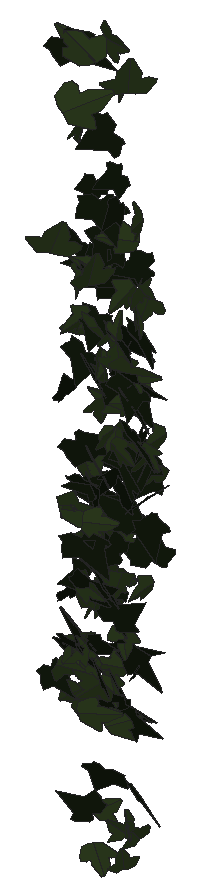
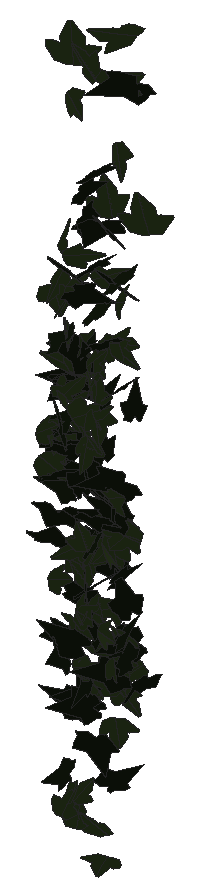
# SketchUp Ruby script. Lengths in inches.
U = 1.inch
M = Sketchup.active_model
def pt(a) = Geom::Point3d.new(a.map { |v| v * U })
def face(e, loops, mat)
  f = e.add_face(loops[0].map { |a| pt(a) })
  loops[1..].each { |l| e.add_face(l.map { |a| pt(a) }).erase! }
  f.material = f.back_material = mat if mat
  f
end
# faces: each face lists its corners as indices into pts; further lists are holes
def faces(e, pts, list, mat = nil) = list.each { |f| face(e, (f[0].is_a?(Array) ? f : [f]).map { |l| l.map { |i| pts[i] } }, mat) }
# xy, xz, yz: faces in a plane at the given z, y or x. An outline is a flat list of corners, or four numbers for a rectangle; further outlines are holes
def ring(l) = l.size == 4 ? [[l[0], l[1]], [l[2], l[1]], [l[2], l[3]], [l[0], l[3]]] : l.each_slice(2).to_a
def flat(e, list, mat, &to3) = list.each { |f| face(e, (f[0].is_a?(Array) ? f : [f]).map { |l| ring(l).map { |u, v| to3.(u, v) } }, mat) }
def xy(e, z, list, mat = nil) = flat(e, list, mat) { |x, y| [x, y, z] }
def xz(e, y, list, mat = nil) = flat(e, list, mat) { |x, z| [x, y, z] }
def yz(e, x, list, mat = nil) = flat(e, list, mat) { |y, z| [x, y, z] }
def lines(e, pts, list) = list.each { |a, b| e.add_line(pt(pts[a]), pt(pts[b])) }
# prism: a flat outline (further loops are holes) pulled along v
def prism(e, loops, v, mat = nil)
  f = face(e, loops, mat); d = Geom::Vector3d.new(v.map { |x| x * U })
  f.pushpull(f.normal.samedirection?(d) ? d.length : -d.length)
end
def box(e, o, s, mat = nil) = prism(e, [[o, [o[0] + s[0], o[1], o[2]], [o[0] + s[0], o[1] + s[1], o[2]], [o[0], o[1] + s[1], o[2]]]], [0, 0, s[2]], mat)
def at(x, y, z, deg = 0) = Geom::Transformation.translation(pt([x, y, z])) * Geom::Transformation.rotation(ORIGIN, Z_AXIS, deg.degrees)
def axes(o, x, y, z) = Geom::Transformation.new([*x, 0, *y, 0, *z, 0, *pt(o).to_a, 1])
def part(name) = M.definitions.add(name)
# library, detail: a bought-in or finely detailed component or shape, given as its bounding box
def library(name, o, s) = part(name).tap { |d| box(d.entities, o, s) }
def detail(e, o, s) = box(e.add_group.entities, o, s)
def put(e, d, t, mat = nil) = e.add_instance(d, t).tap { |i| i.material = mat if mat }
def group(e, t, mat = nil) = e.add_group.tap { |g| g.transformation = t; g.material = mat if mat }.entities
root = M.entities
M.materials.add("1026 AP 7946 SUNNY SIDE UP").color = [254, 231, 186]
M.materials.add("efeu1").color = [18, 25, 13]
M.materials.add("efeu2").color = [43, 57, 29]
c1 = part("ivyleaf_10")
p = [[0,0.5,-0.03],[-0.0625,2.02,-0.43],[-0.19,2.01,-0.46],[-0.54,1.05,-0.29],[-0.52,0.625,-0.18],[-0.83,0.76,-0.28],
  [-1.16,0.64,-0.33],[-1.15,0.33,-0.24],[-0.77,-0.39,0.02],[-0.3,-0.51,0.16],[0.04,-0.48,0.23],[-0.02,2.01,-0.4375],
  [-0.06,2.01,-0.43],[0.04,-0.49,0.23],[0.67,-0.49,0.14],[1.38,0.36,-0.2],[1.375,0.51,-0.24],[0.81,0.65,-0.19],
  [0.62,0.59,-0.15],[0.6,1.09,-0.28],[0.5,1.23,-0.31]]
faces(c1.entities,p,[[0,1,2,3,4,5,6,7,8,9,10],[11,12,0,13,14,15,16,17,18,19,20]],"efeu2")
c2 = part("ivyleaf_9")
p = [[1.54,2.16,1.25],[1.36,2.04,1.19],[-0.21,0.99,0.68],[-0.71,1.11,0.82],[-0.85,0.86,0.67],[-0.8,0.17,0.21],
  [-0.9,-0.01,0.1],[-0.67,-0.16,-0.02],[-0.08,-0.08,-0.05],[-0.03,-0.6,-0.4],[0.65,-0.88,-0.66],[0.83,-0.6,-0.49],
  [1.29,-0.42,-0.43],[1.8125,-0.07,-0.26],[1.21,0.44,0.15]]
faces(c2.entities,p,[[0,1,2,3,4,5,6,7,8,9,10,11,12,13,14]],"efeu1")
put(root,c1,axes([111.49,209.65,262.91],[-0.17375,-0.32185,-0.02419],[-0.02548,-0.01732,0.35033],[-0.50659,0.11126,-0.00932]),"1026 AP 7946 SUNNY SIDE UP")
put(root,c1,axes([111.22,209.35,266.96],[0.25556,0.02321,-0.35537],[0.36802,0.27334,0.1341],[0.4004,-0.26605,0.10356]),"1026 AP 7946 SUNNY SIDE UP")
put(root,c1,axes([110.24,209.98,263.08],[-0.38999,-0.21873,0.04558],[0.02966,0.04722,0.34015],[-0.35003,0.2477,-0.02196]),"1026 AP 7946 SUNNY SIDE UP")
put(root,c1,axes([111.14,209.96,252.59],[0.10276,-0.01725,-0.25564],[0.3866,0.04274,0.06392],[0.05831,-0.25293,0.02671]),"1026 AP 7946 SUNNY SIDE UP")
put(root,c2,axes([111.08,210.48,253.16],[-0.01812,-0.07901,0.2553],[0.02696,-0.2482,-0.082],[0.40878,0.01287,0.01673]),"1026 AP 7946 SUNNY SIDE UP")
put(root,c2,axes([110.69,210.51,255.03],[-0.04185,-0.03352,0.27533],[0.32226,-0.17708,-0.00289],[0.2753,0.20219,0.04524]),"1026 AP 7946 SUNNY SIDE UP")
put(root,c1,axes([110.55,210.51,255.15],[-0.00463,0.00813,0.27853],[0.41593,-0.05615,0.00438],[0.08846,0.26444,-0.00601]),"1026 AP 7946 SUNNY SIDE UP")
put(root,c2,axes([111.0625,210.62,255.24],[0.27088,-0.15391,-0.13249],[0.17626,-0.06532,0.23644],[-0.26045,-0.20427,0.02222]),"1026 AP 7946 SUNNY SIDE UP")
put(root,c2,axes([110.75,210.56,249.9],[0.01042,0.03582,0.25038],[-0.3547,-0.09489,0.02021],[0.15218,-0.22363,0.02995]),"1026 AP 7946 SUNNY SIDE UP")
put(root,c1,axes([110.4,210.61,253.59],[0.33866,-0.13345,-0.08962],[-0.13366,0.02596,-0.25993],[0.21109,0.23054,-0.02079]),"1026 AP 7946 SUNNY SIDE UP")
put(root,c2,axes([110.72,210.8,257.79],[-0.03519,-0.08172,0.27107],[0.08662,-0.26045,-0.0799],[0.4252,0.0463,0.03871]),"1026 AP 7946 SUNNY SIDE UP")
put(root,c2,axes([110.48,210.62,256.1],[-0.08192,-0.17821,-0.20654],[0.1772,0.16968,-0.1855],[0.38144,-0.1171,0.04182]),"1026 AP 7946 SUNNY SIDE UP")
put(root,c1,axes([111.62,210.72,266.97],[-0.3525,-0.27041,-0.0294],[-0.05405,-0.0065,0.36109],[-0.42387,0.22571,-0.0216]),"1026 AP 7946 SUNNY SIDE UP")
put(root,c2,axes([109.98,210.64,253.55],[0.39055,-0.0623,0.07124],[0.09668,-0.03946,-0.26302],[0.11043,0.25489,-0.02169]),"1026 AP 7946 SUNNY SIDE UP")
put(root,c1,axes([111.48,210.74,248.8125],[-0.15422,-0.19699,-0.07207],[-0.06317,-0.05682,0.22612],[-0.32197,0.1055,-0.00984]),"1026 AP 7946 SUNNY SIDE UP")
put(root,c2,axes([111.04,210.66,250.9],[0.22813,0.10021,-0.17766],[-0.21129,-0.10944,-0.18201],[-0.23282,0.19751,-0.0089]),"1026 AP 7946 SUNNY SIDE UP")
put(root,c1,axes([111.39,210.84,249.52],[-0.12943,-0.13186,-0.17606],[-0.1636,-0.13511,0.15892],[-0.29632,0.13219,-0.01084]),"1026 AP 7946 SUNNY SIDE UP")
put(root,c2,axes([109.67,210.66,252.8],[0.08125,-0.16649,-0.18844],[-0.06214,0.17793,-0.17823],[0.38281,0.06422,0.01107]),"1026 AP 7946 SUNNY SIDE UP")
put(root,c2,axes([110.33,210.92,255.01],[-0.10056,-0.07992,0.24078],[-0.18938,-0.20123,-0.10582],[0.33988,-0.13577,0.01228]),"1026 AP 7946 SUNNY SIDE UP")
put(root,c2,axes([110.3125,210.81,253.52],[0.06085,-0.24153,0.12366],[-0.00111,0.12255,0.25213],[-0.42507,-0.03489,0.01704]),"1026 AP 7946 SUNNY SIDE UP")
put(root,c1,axes([109.92,210.64,252.97],[-0.09006,-0.11177,-0.22735],[0.19254,0.18327,-0.12766],[0.33696,-0.13459,0.01218]),"1026 AP 7946 SUNNY SIDE UP")
put(root,c1,axes([111.16,210.9,258.35],[-0.06074,0.01698,-0.25993],[0.27097,-0.18517,-0.04108],[-0.29122,-0.17583,0.01599]),"1026 AP 7946 SUNNY SIDE UP")
put(root,c2,axes([109.82,210.9,259.16],[0.12144,0.12807,0.19805],[-0.17559,-0.15587,0.15286],[0.31687,-0.13546,0.0088]),"1026 AP 7946 SUNNY SIDE UP")
put(root,c1,axes([110.7,210.84,252.69],[-0.34206,-0.03433,0.18124],[-0.2645,-0.05734,-0.22589],[0.09822,-0.27396,0.02287]),"1026 AP 7946 SUNNY SIDE UP")
put(root,c1,axes([110.19,210.85,252.39],[-0.27238,-0.02747,0.15629],[-0.22698,-0.05191,-0.1796],[0.08584,-0.22444,0.02101]),"1026 AP 7946 SUNNY SIDE UP")
put(root,c1,axes([110.57,210.76,256.48],[0.01455,-0.0823,-0.25916],[0.29377,0.17972,-0.05254],[0.29383,-0.17561,0.06536]),"1026 AP 7946 SUNNY SIDE UP")
put(root,c1,axes([109.97,211.09,253.3],[-0.0314,0.05147,0.28562],[0.22525,-0.23721,0.05467],[0.38139,0.14434,-0.00877]),"1026 AP 7946 SUNNY SIDE UP")
put(root,c2,axes([109.91,210.92,254.5],[0.19999,0.20222,0.13212],[-0.12801,-0.09867,0.24508],[0.35307,-0.15032,0.01402]),"1026 AP 7946 SUNNY SIDE UP")
put(root,c2,axes([111.03,211.08,255.78],[-0.0444,0.00518,0.25311],[-0.30761,-0.1501,-0.02079],[0.23379,-0.19651,0.02072]),"1026 AP 7946 SUNNY SIDE UP")
put(root,c2,axes([111.08,210.93,254.29],[-0.14962,0.07109,0.23182],[0.31027,-0.10833,0.1208],[0.20244,0.21858,-0.01381]),"1026 AP 7946 SUNNY SIDE UP")
put(root,c1,axes([111.32,211.125,259.37],[-0.05543,0.07524,0.23947],[0.00636,-0.23422,0.07751],[0.38349,0.01476,0.03333]),"1026 AP 7946 SUNNY SIDE UP")
put(root,c1,axes([111.16,211,255.29],[-0.25373,-0.21656,0.04861],[-0.02158,-0.05001,-0.27786],[0.34826,-0.16088,0.0182]),"1026 AP 7946 SUNNY SIDE UP")
put(root,c1,axes([110.54,211.1,262.2],[0.08727,0.12115,0.215],[-0.16205,-0.18096,0.13585],[0.34207,-0.11664,0.0095]),"1026 AP 7946 SUNNY SIDE UP")
put(root,c1,axes([111.31,211.03,249.77],[-0.08271,0.2066,-0.07727],[0.02138,-0.07513,-0.22001],[-0.34558,-0.0541,0.00488]),"1026 AP 7946 SUNNY SIDE UP")
put(root,c1,axes([110.03,211.21,260.87],[-0.01886,-0.08661,0.27005],[0.01863,-0.2628,-0.09026],[0.43444,0.00751,0.0156]),"1026 AP 7946 SUNNY SIDE UP")
put(root,c1,axes([109.96,211.22,261.89],[-0.00643,-0.13249,0.26396],[0.22055,-0.22564,-0.11887],[0.39752,0.12304,0.07022]),"1026 AP 7946 SUNNY SIDE UP")
put(root,c1,axes([111.49,211.18,249.29],[-0.12051,-0.16603,-0.17776],[-0.1047,-0.15822,0.18741],[-0.36056,0.10144,0.00499]),"1026 AP 7946 SUNNY SIDE UP")
put(root,c2,axes([111.3,211.19,259.76],[-0.10665,-0.25601,0.02651],[0.00151,-0.02837,-0.27288],[0.40482,-0.06734,0.008]),"1026 AP 7946 SUNNY SIDE UP")
put(root,c2,axes([111.02,211.18,257.08],[-0.01672,0.01143,0.28467],[0.14094,-0.2614,0.01317],[0.41129,0.09004,0.00706]),"1026 AP 7946 SUNNY SIDE UP")
put(root,c1,axes([111.16,211.26,261.84],[-0.08169,-0.12417,0.26344],[0.06008,-0.26133,-0.12392],[0.44393,0.01252,0.06525]),"1026 AP 7946 SUNNY SIDE UP")
put(root,c2,axes([111.15,211.21,259.46],[0.1959,-0.226,0.12777],[0.06796,-0.11893,-0.26594],[0.40062,0.13069,-0.01737]),"1026 AP 7946 SUNNY SIDE UP")
put(root,c1,axes([110.25,211.09,254.49],[-0.24127,0.0035,-0.17969],[0.26911,-0.04217,-0.1562],[-0.05337,-0.22846,0.0247]),"1026 AP 7946 SUNNY SIDE UP")
put(root,c2,axes([111.3,211.23,258.59],[0.17591,-0.23109,0.1151],[0.07346,-0.10297,-0.26508],[0.39778,0.12121,-0.00195]),"1026 AP 7946 SUNNY SIDE UP")
put(root,c2,axes([111.45,211.1875,258.25],[-0.19051,-0.2117,-0.09954],[0.11214,0.0685,-0.24945],[0.34748,-0.13817,0.02593]),"1026 AP 7946 SUNNY SIDE UP")
put(root,c1,axes([110.25,211.02,255.96],[-0.23597,-0.14918,-0.17363],[0.22523,0.09165,-0.21551],[0.27171,-0.20553,0.02785]),"1026 AP 7946 SUNNY SIDE UP")
put(root,c2,axes([110.23,211.25,256.7],[-0.06616,0.04582,0.27342],[0.04861,-0.26577,0.05082],[0.42029,0.03795,0.03716]),"1026 AP 7946 SUNNY SIDE UP")
put(root,c2,axes([111.34,211.17,253.48],[-0.02862,-0.03952,-0.2682],[0.3987,0.06693,-0.02836],[0.11037,-0.25202,0.03291]),"1026 AP 7946 SUNNY SIDE UP")
put(root,c1,axes([110.29,211.15,260.74],[-0.20627,-0.01504,0.25226],[-0.36961,-0.07214,-0.13467],[0.11092,-0.26834,0.02037]),"1026 AP 7946 SUNNY SIDE UP")
put(root,c1,axes([110.28,211.15,253.01],[0.32252,-0.11888,-0.08315],[-0.126,0.02071,-0.24314],[0.18683,0.2192,-0.02045]),"1026 AP 7946 SUNNY SIDE UP")
put(root,c2,axes([111.38,211.25,258.07],[-0.27406,-0.23299,-0.08552],[0.10022,0.05415,-0.29887],[0.37506,-0.18472,0.01737]),"1026 AP 7946 SUNNY SIDE UP")
put(root,c1,axes([110.92,211.09,251.76],[0.2379,-0.01681,-0.20773],[0.31792,0.01842,0.15489],[0.00739,-0.25134,0.02376]),"1026 AP 7946 SUNNY SIDE UP")
put(root,c2,axes([110.84,211.32,263.69],[0.00225,-0.02976,-0.25435],[0.22669,-0.20087,0.02465],[-0.31829,-0.14327,0.01576]),"1026 AP 7946 SUNNY SIDE UP")
put(root,c2,axes([111.01,211.17,257.625],[-0.04955,0.2018,-0.19039],[0.04198,-0.18404,-0.21149],[-0.42945,-0.04128,0.0013]),"1026 AP 7946 SUNNY SIDE UP")
put(root,c2,axes([110.58,211.14,262.33],[-0.31313,0.10686,0.10333],[-0.15563,0.02537,-0.23154],[-0.16909,-0.22126,0.02174]),"1026 AP 7946 SUNNY SIDE UP")
put(root,c1,axes([109.74,211.09,256.36],[-0.07481,-0.00181,0.29244],[0.41046,0.11285,0.04648],[-0.17544,0.2648,-0.01597]),"1026 AP 7946 SUNNY SIDE UP")
put(root,c1,axes([110.79,211.23,258.4],[0.34128,-0.11553,0.09189],[0.10535,-0.06446,-0.25248],[0.2046,0.22589,-0.02327]),"1026 AP 7946 SUNNY SIDE UP")
put(root,c1,axes([110.06,211.13,265.42],[0.01673,-0.28303,-0.07759],[-0.00579,0.07362,-0.29135],[0.45984,0.01122,-0.00085]),"1026 AP 7946 SUNNY SIDE UP")
put(root,c2,axes([110.68,211.11,252.21],[0.3168,-0.00602,0.15531],[0.23349,-0.03696,-0.20613],[0.04232,0.24892,-0.02536]),"1026 AP 7946 SUNNY SIDE UP")
put(root,c2,axes([109.84,211.36,262.4375],[0.01033,-0.23764,0.16501],[0.05479,-0.15972,-0.24447],[0.44848,0.02498,0.02607]),"1026 AP 7946 SUNNY SIDE UP")
put(root,c1,axes([109.89,211.15,256.34],[-0.3147,-0.05783,-0.12673],[0.20194,-0.01044,-0.21081],[0.0686,-0.23452,0.03918]),"1026 AP 7946 SUNNY SIDE UP")
put(root,c2,axes([111.125,211.2,251.93],[0.19868,-0.04522,-0.22264],[0.33768,0.08185,0.11232],[0.07893,-0.23635,0.07989]),"1026 AP 7946 SUNNY SIDE UP")
put(root,c1,axes([111.0625,211.22,253.87],[0.35574,-0.04589,0.09332],[0.13225,-0.0404,-0.23704],[0.09012,0.24043,-0.02052]),"1026 AP 7946 SUNNY SIDE UP")
put(root,c1,axes([110.47,211.28,260.09],[0.02045,0.17407,-0.17279],[-0.01664,-0.16839,-0.1808],[-0.38081,0.01671,-0.00138]),"1026 AP 7946 SUNNY SIDE UP")
put(root,c1,axes([111.64,211.23,258.1],[0.03648,-0.27948,0.01841],[-0.00074,-0.01956,-0.28902],[0.44052,0.02311,-0.00201]),"1026 AP 7946 SUNNY SIDE UP")
put(root,c1,axes([111.51,211.17,258.34],[-0.33097,-0.01592,-0.13266],[0.20375,-0.017,-0.21628],[0.00733,-0.24612,0.02207]),"1026 AP 7946 SUNNY SIDE UP")
put(root,c2,axes([109.91,211.39,259.89],[-0.0869,-0.24525,0.12096],[-0.02637,-0.11794,-0.25953],[0.42769,-0.0571,0.00858]),"1026 AP 7946 SUNNY SIDE UP")
put(root,c1,axes([110.14,211.21,267.01],[0.31464,0.15867,0.20981],[-0.29848,-0.08256,0.25907],[0.2735,-0.27264,0.04137]),"1026 AP 7946 SUNNY SIDE UP")
put(root,c2,axes([110.42,211.25,259.41],[0.10666,-0.20688,0.1086],[-0.02864,0.10596,0.22444],[-0.36482,-0.0688,0.01413]),"1026 AP 7946 SUNNY SIDE UP")
put(root,c1,axes([110.65,211.29,252.6],[0.29472,-0.03992,0.15096],[0.21449,-0.05891,-0.19631],[0.10579,0.23065,-0.02254]),"1026 AP 7946 SUNNY SIDE UP")
put(root,c2,axes([111.35,211.28,258.19],[0.00005,0.18334,0.21946],[-0.03407,-0.21136,0.18707],[0.43938,-0.01641,0.01448]),"1026 AP 7946 SUNNY SIDE UP")
put(root,c2,axes([110.8,211.43,264.33],[0.02707,-0.12069,-0.22378],[0.13537,-0.20064,0.12108],[-0.36554,-0.08324,0.02827]),"1026 AP 7946 SUNNY SIDE UP")
put(root,c2,axes([111.28,211.28,250.28],[0.26725,-0.18035,0.02517],[0.0105,-0.02863,-0.25502],[0.2862,0.16946,-0.01415]),"1026 AP 7946 SUNNY SIDE UP")
put(root,c2,axes([110.28,211.38,260.88],[-0.17114,-0.22907,0.01658],[0.00197,-0.01984,-0.2612],[0.36122,-0.10842,0.00928]),"1026 AP 7946 SUNNY SIDE UP")
put(root,c1,axes([111.4,211.28,261.42],[-0.06478,0.22319,-0.09514],[0.01573,-0.09331,-0.23426],[-0.38024,-0.04188,0.00652]),"1026 AP 7946 SUNNY SIDE UP")
put(root,c2,axes([111.08,211.22,259.6],[-0.11412,-0.14165,-0.24682],[0.22292,0.19329,-0.16139],[0.37535,-0.15787,0.02081]),"1026 AP 7946 SUNNY SIDE UP")
put(root,c1,axes([110.87,211.34,252.96],[0.02811,0.03256,0.23361],[-0.24508,-0.16471,0.03609],[0.26361,-0.15661,0.00864]),"1026 AP 7946 SUNNY SIDE UP")
put(root,c2,axes([110.4375,211.23,257.09],[-0.30221,0.127,0.08398],[-0.12358,0.02709,-0.23631],[-0.20187,-0.20672,0.01894]),"1026 AP 7946 SUNNY SIDE UP")
put(root,c1,axes([110.18,211.38,256.06],[0.13797,-0.22143,0.15398],[0.09009,-0.13942,-0.24618],[0.41144,0.10478,0.00227]),"1026 AP 7946 SUNNY SIDE UP")
put(root,c2,axes([110.44,211.28,263.62],[-0.11434,-0.23654,-0.16304],[0.06959,0.15056,-0.25405],[0.44088,-0.08511,-0.00218]),"1026 AP 7946 SUNNY SIDE UP")
put(root,c1,axes([111.0625,211.2,259.89],[-0.14489,-0.02792,0.2898],[0.40382,0.11578,0.09913],[-0.18636,0.27259,-0.01052]),"1026 AP 7946 SUNNY SIDE UP")
put(root,c1,axes([110.32,211.24,248.55],[0.28448,0.15464,0.06083],[0.08774,0.02399,-0.24438],[-0.24452,0.18852,-0.01693]),"1026 AP 7946 SUNNY SIDE UP")
put(root,c2,axes([110.97,211.22,259.71],[0.28205,-0.01547,0.17128],[0.25628,-0.03743,-0.18486],[0.05772,0.24176,-0.01621]),"1026 AP 7946 SUNNY SIDE UP")
put(root,c1,axes([110.88,211.29,260.02],[-0.32415,-0.13251,-0.02107],[-0.0432,0.00643,0.25165],[-0.20618,0.20699,-0.0196]),"1026 AP 7946 SUNNY SIDE UP")
put(root,c2,axes([109.64,211.15,267.1875],[0.05033,-0.07104,-0.30296],[0.19484,0.27243,-0.05238],[0.43331,-0.11425,0.05874]),"1026 AP 7946 SUNNY SIDE UP")
put(root,c2,axes([110.72,211.41,260.59],[0.09821,-0.20034,0.14621],[0.09042,-0.13164,-0.21654],[0.37638,0.0839,0.01387]),"1026 AP 7946 SUNNY SIDE UP")
put(root,c1,axes([109.96,211.32,253.34],[-0.14383,-0.23715,0.05455],[-0.01202,-0.05518,-0.26186],[0.38236,-0.09094,0.01228]),"1026 AP 7946 SUNNY SIDE UP")
put(root,c2,axes([111.15,211.32,256.49],[-0.28146,-0.16337,-0.08115],[-0.09836,-0.04688,0.24928],[-0.26701,0.18948,-0.00629]),"1026 AP 7946 SUNNY SIDE UP")
put(root,c1,axes([110.49,211.28,259.52],[-0.33827,0.12401,0.0465],[0.07536,-0.00558,0.25504],[0.19293,0.2196,-0.01808]),"1026 AP 7946 SUNNY SIDE UP")
put(root,c1,axes([110.78,211.33,255.06],[-0.17014,0.04305,0.23472],[0.35129,-0.04695,0.1183],[0.09619,0.2476,-0.01684]),"1026 AP 7946 SUNNY SIDE UP")
put(root,c2,axes([110.53,211.51,262.62],[-0.15861,-0.22863,0.17006],[-0.08469,-0.15788,-0.25806],[0.43647,-0.11371,0.01173]),"1026 AP 7946 SUNNY SIDE UP")
put(root,c1,axes([111.28,211.45,259.52],[0.05563,-0.2115,0.2039],[0.06807,-0.19452,-0.22191],[0.45167,0.05537,0.00833]),"1026 AP 7946 SUNNY SIDE UP")
put(root,c2,axes([110.52,211.49,255.92],[-0.02811,-0.12492,0.23976],[-0.00921,-0.23373,-0.13068],[0.41621,-0.01361,0.0133]),"1026 AP 7946 SUNNY SIDE UP")
put(root,c1,axes([110.08,211.17,252.67],[0.21601,0.04412,-0.20897],[0.26983,0.11327,0.14559],[0.18437,-0.21747,0.03176]),"1026 AP 7946 SUNNY SIDE UP")
put(root,c2,axes([109.54,211.39,253.61],[0.22731,-0.17348,0.10559],[0.08468,-0.08954,-0.23268],[0.30612,0.15359,-0.01404]),"1026 AP 7946 SUNNY SIDE UP")
put(root,c2,axes([111.46,211.12,257],[-0.05208,0.22311,-0.10885],[-0.01816,0.10637,0.23295],[0.38861,0.03487,-0.0037]),"1026 AP 7946 SUNNY SIDE UP")
put(root,c2,axes([109.8,211.3,256.84],[0.27555,0.04265,-0.16549],[0.22911,0.07361,0.18403],[0.1265,-0.22622,0.02717]),"1026 AP 7946 SUNNY SIDE UP")
put(root,c1,axes([109.97,211.33,251.93],[-0.28297,-0.1602,0.02948],[-0.01583,-0.03298,-0.24772],[0.25564,-0.17936,0.01729]),"1026 AP 7946 SUNNY SIDE UP")
put(root,c2,axes([110.99,211.27,253.41],[0.29331,0.09223,-0.13751],[0.16268,0.09009,0.21276],[0.19741,-0.21128,0.02899]),"1026 AP 7946 SUNNY SIDE UP")
put(root,c1,axes([110.58,211.15,254.5],[-0.04235,-0.1547,-0.24127],[0.11402,0.22254,-0.15933],[0.42516,-0.07509,0.01869]),"1026 AP 7946 SUNNY SIDE UP")
put(root,c1,axes([110.5,211.31,259.03],[-0.11722,-0.28072,-0.03145],[0.01324,0.0277,-0.29905],[0.44354,-0.07501,0.00062]),"1026 AP 7946 SUNNY SIDE UP")
put(root,c1,axes([111.58,211.36,261.66],[-0.32275,-0.12853,0.06004],[-0.06205,-0.04783,-0.249],[0.21356,-0.20815,0.0184]),"1026 AP 7946 SUNNY SIDE UP")
put(root,c2,axes([110.67,211.27,252.07],[0.30997,0.01065,0.15168],[0.232,-0.01794,-0.20236],[0.00351,0.24536,-0.01993]),"1026 AP 7946 SUNNY SIDE UP")
put(root,c2,axes([110.79,211.47,254.8],[-0.03001,-0.25074,-0.0431],[-0.00826,-0.04013,0.25882],[-0.39927,0.01968,-0.00212]),"1026 AP 7946 SUNNY SIDE UP")
put(root,c1,axes([110.82,211.45,259.02],[-0.2014,-0.03972,-0.24725],[-0.34857,-0.09203,0.13716],[-0.15668,0.25579,0.01268]),"1026 AP 7946 SUNNY SIDE UP")
put(root,c2,axes([110.51,211.45,254.29],[-0.03525,-0.02507,-0.25831],[0.39527,-0.0175,-0.02147],[-0.02404,-0.25098,0.0258]),"1026 AP 7946 SUNNY SIDE UP")
put(root,c1,axes([111.49,211.24,261.99],[-0.01729,-0.21845,-0.19933],[0.11415,0.18424,-0.21887],[0.4431,-0.05599,0.04861]),"1026 AP 7946 SUNNY SIDE UP")
put(root,c2,axes([110.67,211.33,252.75],[0.28268,-0.12997,-0.1275],[-0.17706,0.05338,-0.2273],[0.2187,0.2112,-0.01923]),"1026 AP 7946 SUNNY SIDE UP")
put(root,c1,axes([111.42,211.55,254.95],[-0.001,-0.07393,0.24081],[0.04135,-0.23285,-0.07702],[0.38391,0.02489,0.00892]),"1026 AP 7946 SUNNY SIDE UP")
put(root,c1,axes([110.67,211.4,260.36],[0.15316,-0.22395,-0.01418],[-0.02208,0.00751,-0.25134],[0.352,0.09792,-0.00959]),"1026 AP 7946 SUNNY SIDE UP")
put(root,c2,axes([110.45,211.49,256.73],[-0.33162,-0.13176,-0.07817],[0.11869,0.02043,-0.25509],[0.20687,-0.22295,0.02105]),"1026 AP 7946 SUNNY SIDE UP")
put(root,c1,axes([110.48,211.48,267.3125],[-0.16531,0.04716,0.30102],[0.42779,-0.10598,0.11795],[0.1822,0.29162,-0.00383]),"1026 AP 7946 SUNNY SIDE UP")
put(root,c2,axes([110.85,211.54,261.98],[-0.01785,-0.04666,-0.24818],[-0.06601,-0.23697,0.04799],[-0.37974,0.04339,0.00333]),"1026 AP 7946 SUNNY SIDE UP")
put(root,c2,axes([111.45,211.46,256.53],[-0.24013,-0.11611,-0.19712],[0.28083,0.07508,-0.19402],[0.21063,-0.23248,0.03396]),"1026 AP 7946 SUNNY SIDE UP")
put(root,c1,axes([110.74,211.4,255.95],[-0.17741,-0.20061,0.02408],[0.00855,0.02505,0.23713],[-0.31767,0.11271,-0.00707]),"1026 AP 7946 SUNNY SIDE UP")
put(root,c2,axes([111.13,211.51,258.19],[-0.23067,-0.20218,-0.05295],[0.06776,0.03068,-0.25659],[0.32049,-0.152,0.01614]),"1026 AP 7946 SUNNY SIDE UP")
put(root,c1,axes([110.71,211.58,254.45],[0.0722,-0.06769,0.25639],[0.14291,-0.23274,-0.08372],[0.38015,0.10035,-0.01722]),"1026 AP 7946 SUNNY SIDE UP")
put(root,c2,axes([110.31,211.61,261.59],[-0.10483,-0.15152,0.21878],[0.01044,-0.22095,-0.1609],[0.41117,-0.03302,0.05986]),"1026 AP 7946 SUNNY SIDE UP")
put(root,c1,axes([110.76,211.24,259.81],[-0.01393,0.06069,0.2435],[-0.26313,0.17018,-0.05056],[-0.27857,-0.16378,0.03558]),"1026 AP 7946 SUNNY SIDE UP")
put(root,c1,axes([110.94,211.56,262.8],[-0.0256,0.07147,0.2582],[-0.19869,-0.22135,0.05537],[0.35772,-0.11783,0.04923]),"1026 AP 7946 SUNNY SIDE UP")
put(root,c1,axes([110.69,211.35,258.33],[-0.09514,-0.25953,-0.14075],[0.06846,0.12849,-0.27351],[0.45498,-0.0736,0.01172]),"1026 AP 7946 SUNNY SIDE UP")
put(root,c1,axes([110.81,211.28,260.67],[0.01678,0.17216,-0.17604],[0.02392,0.17122,0.17867],[0.38176,-0.0183,-0.00346]),"1026 AP 7946 SUNNY SIDE UP")
put(root,c1,axes([110.37,211.6,260.46],[-0.02298,0.08437,0.24322],[0.0665,-0.23179,0.08685],[0.38786,0.04474,-0.00048]),"1026 AP 7946 SUNNY SIDE UP")
put(root,c2,axes([111.47,211.45,262.41],[-0.34263,0.1043,0.06112],[-0.10297,-0.00175,-0.24708],[-0.15755,-0.22567,0.02856]),"1026 AP 7946 SUNNY SIDE UP")
put(root,c1,axes([111.625,211.58,257.7],[-0.15174,-0.17932,0.18775],[-0.08809,-0.17634,-0.20917],[0.39343,-0.10864,0.02558]),"1026 AP 7946 SUNNY SIDE UP")
put(root,c1,axes([110.625,211.59,254.41],[-0.07791,-0.13907,0.19611],[-0.06581,-0.18706,-0.15247],[0.36583,-0.06327,0.01433]),"1026 AP 7946 SUNNY SIDE UP")
put(root,c1,axes([111.16,211.46,259.41],[0.20905,0.22218,0.10092],[-0.10202,-0.07364,0.26575],[0.36711,-0.14699,0.01638]),"1026 AP 7946 SUNNY SIDE UP")
put(root,c1,axes([111.27,211.35,260.96],[0.06367,-0.17904,-0.17241],[-0.06224,0.16158,-0.18814],[0.3792,0.05658,-0.00193]),"1026 AP 7946 SUNNY SIDE UP")
put(root,c2,axes([111.17,211.62,260.7],[0.08472,-0.22891,0.1383],[0.06401,-0.12958,-0.24286],[0.41338,0.06698,0.00926]),"1026 AP 7946 SUNNY SIDE UP")
put(root,c2,axes([109.77,211.38,257.78],[0.05644,-0.05391,-0.28653],[0.27216,0.22575,-0.02077],[0.35207,-0.16587,0.06199]),"1026 AP 7946 SUNNY SIDE UP")
put(root,c1,axes([110.07,211.38,257.26],[0.31411,-0.03916,0.21418],[-0.30601,0.07889,0.20819],[-0.13133,-0.27749,0.02717]),"1026 AP 7946 SUNNY SIDE UP")
put(root,c2,axes([111.4,211.64,257.49],[-0.21786,-0.19091,0.077],[-0.04802,-0.07131,-0.24284],[0.31941,-0.14093,0.01601]),"1026 AP 7946 SUNNY SIDE UP")
put(root,c2,axes([109.9,211.35,253.18],[0.09279,0.07648,-0.23682],[0.17665,0.20148,0.09976],[0.33823,-0.12621,0.01286]),"1026 AP 7946 SUNNY SIDE UP")
put(root,c2,axes([110.55,211.62,255.22],[-0.05512,-0.01361,-0.25236],[0.33996,-0.11851,-0.02579],[-0.18209,-0.21715,0.02824]),"1026 AP 7946 SUNNY SIDE UP")
put(root,c2,axes([111.36,211.28,253.05],[0.07852,0.09082,0.23461],[0.12218,0.21402,-0.10446],[-0.36485,0.09121,0.01551]),"1026 AP 7946 SUNNY SIDE UP")
put(root,c2,axes([110.02,211.61,263.81],[-0.26718,-0.0476,-0.17456],[0.27611,-0.05551,-0.16593],[-0.01119,-0.23326,0.07361]),"1026 AP 7946 SUNNY SIDE UP")
put(root,c1,axes([110.08,211.63,254.18],[0.07039,-0.15658,0.16963],[0.05071,-0.16266,-0.16843],[0.35469,0.05433,-0.00958]),"1026 AP 7946 SUNNY SIDE UP")
put(root,c1,axes([110.85,211.32,255.87],[-0.11151,-0.0981,-0.2811],[0.28484,0.20361,-0.12298],[0.35494,-0.19422,0.01038]),"1026 AP 7946 SUNNY SIDE UP")
put(root,c1,axes([110.93,211.59,266.56],[0.03557,-0.24746,0.08631],[0.01956,-0.08439,-0.25645],[0.41106,0.02543,0.00473]),"1026 AP 7946 SUNNY SIDE UP")
put(root,c1,axes([111.64,211.69,258.43],[-0.01872,-0.01595,0.26741],[0.08532,-0.25437,-0.01502],[0.40006,0.0535,0.01572]),"1026 AP 7946 SUNNY SIDE UP")
put(root,c2,axes([111.65,211.4,255.72],[-0.41992,-0.01072,0.0773],[0.11569,0.03026,0.27419],[-0.02902,0.27576,-0.02544]),"1026 AP 7946 SUNNY SIDE UP")
put(root,c1,axes([110.24,211.46,249.36],[0.25877,-0.0251,-0.15386],[0.23754,0.01507,0.16913],[-0.01315,-0.22162,0.0276]),"1026 AP 7946 SUNNY SIDE UP")
put(root,c2,axes([110.33,211.75,265],[-0.22727,-0.14848,0.23157],[-0.16185,-0.20632,-0.209],[0.39266,-0.17098,0.04789]),"1026 AP 7946 SUNNY SIDE UP")
put(root,c2,axes([110.62,211.55,260.56],[0.13701,0.00123,-0.26247],[0.39095,0.05844,0.08823],[0.08757,-0.26286,0.01677]),"1026 AP 7946 SUNNY SIDE UP")
put(root,c1,axes([111.07,211.72,263.2],[-0.08951,0.07388,0.29585],[0.22135,-0.25015,0.09372],[0.40964,0.15131,0.01401]),"1026 AP 7946 SUNNY SIDE UP")
